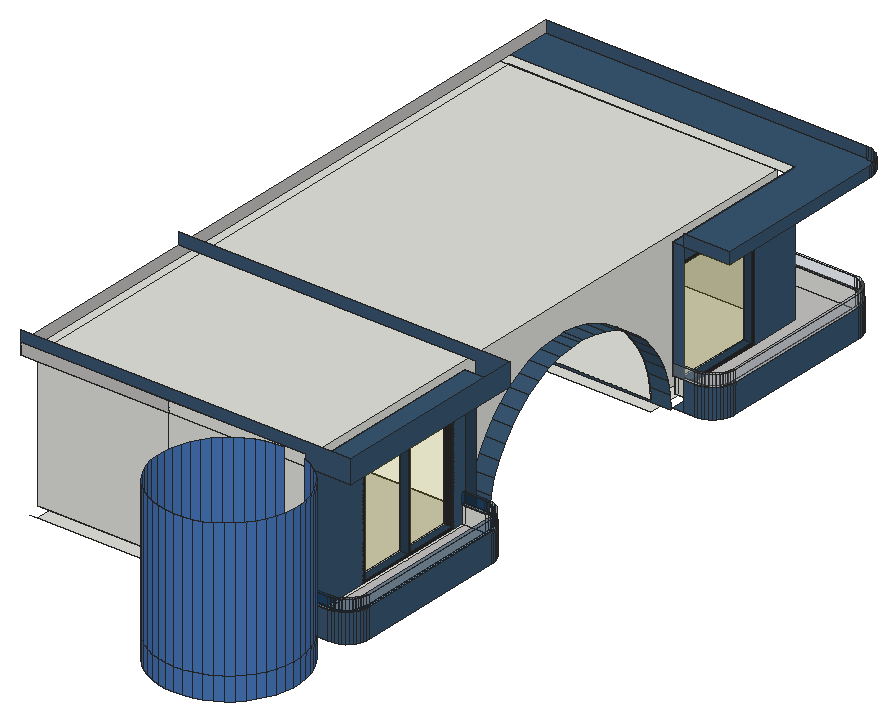
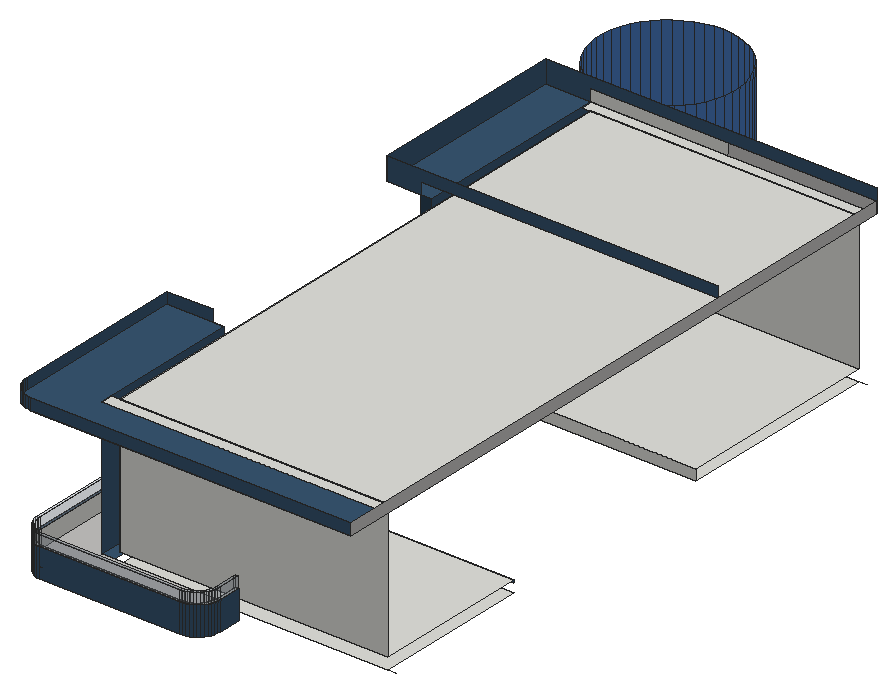
# SketchUp Ruby script. Lengths in inches.
U = 1.inch
M = Sketchup.active_model
def pt(a) = Geom::Point3d.new(a.map { |v| v * U })
def face(e, loops, mat)
  f = e.add_face(loops[0].map { |a| pt(a) })
  loops[1..].each { |l| e.add_face(l.map { |a| pt(a) }).erase! }
  f.material = f.back_material = mat if mat
  f
end
# faces: each face lists its corners as indices into pts; further lists are holes
def faces(e, pts, list, mat = nil) = list.each { |f| face(e, (f[0].is_a?(Array) ? f : [f]).map { |l| l.map { |i| pts[i] } }, mat) }
# xy, xz, yz: faces in a plane at the given z, y or x. An outline is a flat list of corners, or four numbers for a rectangle; further outlines are holes
def ring(l) = l.size == 4 ? [[l[0], l[1]], [l[2], l[1]], [l[2], l[3]], [l[0], l[3]]] : l.each_slice(2).to_a
def flat(e, list, mat, &to3) = list.each { |f| face(e, (f[0].is_a?(Array) ? f : [f]).map { |l| ring(l).map { |u, v| to3.(u, v) } }, mat) }
def xy(e, z, list, mat = nil) = flat(e, list, mat) { |x, y| [x, y, z] }
def xz(e, y, list, mat = nil) = flat(e, list, mat) { |x, z| [x, y, z] }
def yz(e, x, list, mat = nil) = flat(e, list, mat) { |y, z| [x, y, z] }
def lines(e, pts, list) = list.each { |a, b| e.add_line(pt(pts[a]), pt(pts[b])) }
# prism: a flat outline (further loops are holes) pulled along v
def prism(e, loops, v, mat = nil)
  f = face(e, loops, mat); d = Geom::Vector3d.new(v.map { |x| x * U })
  f.pushpull(f.normal.samedirection?(d) ? d.length : -d.length)
end
def box(e, o, s, mat = nil) = prism(e, [[o, [o[0] + s[0], o[1], o[2]], [o[0] + s[0], o[1] + s[1], o[2]], [o[0], o[1] + s[1], o[2]]]], [0, 0, s[2]], mat)
def at(x, y, z, deg = 0) = Geom::Transformation.translation(pt([x, y, z])) * Geom::Transformation.rotation(ORIGIN, Z_AXIS, deg.degrees)
def axes(o, x, y, z) = Geom::Transformation.new([*x, 0, *y, 0, *z, 0, *pt(o).to_a, 1])
def part(name) = M.definitions.add(name)
# library, detail: a bought-in or finely detailed component or shape, given as its bounding box
def library(name, o, s) = part(name).tap { |d| box(d.entities, o, s) }
def detail(e, o, s) = box(e.add_group.entities, o, s)
def put(e, d, t, mat = nil) = e.add_instance(d, t).tap { |i| i.material = mat if mat }
def group(e, t, mat = nil) = e.add_group.tap { |g| g.transformation = t; g.material = mat if mat }.entities
root = M.entities
M.materials.add("Carpet_01_1K").color = [196, 195, 193]
M.materials.add("Carpet_04_1K").color = [56, 85, 112]
M.materials.add("Carpet_04_1K1").color = [43, 65, 85]
M.materials.add("Glass_Basic_01").color = [186, 175, 28]
M.materials["Glass_Basic_01"].alpha = 0.25
M.materials.add("Glass_Basic_1").color = [0, 47, 91]
M.materials["Glass_Basic_1"].alpha = 0.25
M.materials.add("Glass_Basic_2").color = [161, 173, 186]
M.materials["Glass_Basic_2"].alpha = 0.25
M.materials.add("Glass_Mirror_01").color = [71, 118, 185]
M.materials.add("ThomThom - Buttons2").color = [40, 40, 43]
c1 = part("Group\#1")
prism(c1.entities,[[[0,206.04,0],[0,209.04,0],[24,209.04,0],[24.001,209.04,0],[27.133,208.835,0],[30.212,208.222,0],[33.184,207.213,0],[36,205.825,0],[38.61,204.081,0],[40.971,202.011,0],[43.04,199.65,0],[44.785,197.04,0],[46.173,194.224,0],[47.182,191.252,0],[47.795,188.173,0],[48,185.04,0],[48,24,0],[47.795,20.867,0],[47.182,17.788,0],[46.602,16.08,0],[46.173,14.816,0],[44.785,12,0],[43.04,9.39,0],[40.971,7.029,0],[38.61,4.96,0],[36,3.215,0],[33.184,1.827,0],[30.212,0.818,0],[27.133,0.205,0],[24,0,0],[0,0,0],[0,3,0],[3,3,0],[24,3,0],[26.741,3.18,0],[29.435,3.716,0],[32.036,4.599,0],[34.5,5.814,0],[36.784,7.34,0],[38.849,9.151,0],[40.66,11.216,0],[42.187,13.5,0],[43.401,15.964,0],[44.284,18.565,0],[44.82,21.259,0],[45,24,0],[45,185.04,0],[44.82,187.781,0],[44.284,190.475,0],[43.401,193.076,0],[42.187,195.54,0],[40.66,197.824,0],[38.849,199.889,0],[36.784,201.701,0],[34.5,203.227,0],[32.036,204.442,0],[29.435,205.325,0],[26.741,205.86,0],[24,206.04,0],[3,206.04,0]]],[0,0,12])
c2 = part("Group\#2")
prism(c2.entities,[[[147,3,0],[168,3,0],[170.74,3.18,0],[173.44,3.72,0],[176.04,4.6,0],[178.5,5.8125,0],[180.78,7.34,0],[182.85,9.15,0],[184.66,11.22,0],[186.1875,13.5,0],[187.4,15.96,0],[188.28,18.56,0],[188.82,21.26,0],[189,24,0],[189,184.94,0],[188.8125,187.78,0],[188.28,190.47,0],[187.4,193.07,0],[186.18,195.54,0],[184.66,197.82,0],[182.84,199.88,0],[180.78,201.7,0],[178.5,203.22,0],[176.03,204.4375,0],[173.43,205.32,0],[171.01,205.8,0],[24,205.8,0],[21.26,205.62,0],[18.56,205.08,0],[15.96,204.2,0],[13.5,202.99,0],[11.22,201.46,0],[9.15,199.65,0],[7.34,197.58,0],[5.8125,195.3,0],[4.6,192.84,0],[3.72,190.24,0],[3.18,187.54,0],[3,184.8,0],[3,163.8,0],[3,160.8,0],[0,160.8,0],[0,184.8,0],[0.21,187.93,0],[0.82,191.01,0],[1.83,193.98,0],[3.22,196.8,0],[4.96,199.41,0],[7.03,201.77,0],[9.39,203.84,0],[12,205.58,0],[14.82,206.97,0],[17.79,207.98,0],[20.87,208.59,0],[24,208.8,0],[171.31,208.8,0],[174.21,208.22,0],[177.18,207.21,0],[180,205.82,0],[182.61,204.08,0],[184.97,202.01,0],[187.04,199.65,0],[188.78,197.04,0],[190.17,194.22,0],[191.18,191.25,0],[191.79,188.17,0],[192,185.04,0],[192,24,0],[191.79,20.87,0],[191.18,17.79,0],[190.17,14.82,0],[188.78,12,0],[187.04,9.39,0],[184.97,7.03,0],[182.61,4.96,0],[180,3.22,0],[177.18,1.83,0],[174.21,0.82,0],[171.13,0.21,0],[168,0,0],[144,0,0],[144,3,0]]],[0,0,12])
xy(root,1230,[[39.57,167.5625,321.57,381.51],[39.57,620.85,321.57,786.64]])
xy(root,1230,[[330.57,155.5,330.57,364.54,354.57,364.54,357.71,364.34,360.79,363.72,363.76,362.71,366.57,361.33,369.19,359.58,371.55,357.51,373.62,355.15,375.36,352.54,376.75,349.73,377.76,346.75,378.37,343.67,378.57,340.54,378.57,179.5,378.37,176.37,377.76,173.29,376.75,170.32,375.36,167.5,373.62,164.89,371.55,162.53,369.19,160.46,366.57,158.72,363.76,157.33,360.79,156.32,357.71,155.71,354.57,155.5],[330.57,637.9,330.57,798.7,186.57,798.7,186.57,822.7,186.78,825.83,187.39,828.91,188.4,831.89,189.79,834.7,191.53,837.3125,193.6,839.67,195.96,841.74,198.57,843.49,201.39,844.875,204.36,845.88,207.44,846.5,210.57,846.7,357.88,846.7,360.79,846.12,363.76,845.11,366.57,843.73,369.19,841.98,371.55,839.91,373.62,837.55,375.36,834.94,376.75,832.125,377.76,829.15,378.37,826.07,378.57,822.94,378.57,661.9,378.37,658.77,377.76,655.6875,376.75,652.72,375.36,649.9,373.62,647.29,371.55,644.93,369.19,642.86,366.57,641.12,363.76,639.73,360.79,638.72,357.71,638.11,354.57,637.9]],"Carpet_04_1K")
xy(root,1242,[[330.57,158.5,333.57,361.54],[39.57,167.5625,321.57,381.59],[39.57,620.93,321.57,786.64]])
xy(root,1242,[[333.57,158.5,354.57,158.5,357.32,158.68,360.01,159.22,362.61,160.1,365.07,161.31,367.36,162.84,369.42,164.65,371.24,166.72,372.76,169,373.98,171.46,374.86,174.07,375.4,176.76,375.57,179.5,375.57,340.54,375.4,343.28,374.86,345.98,373.98,348.58,372.76,351.04,371.24,353.33,369.42,355.39,367.36,357.2,365.07,358.73,362.61,359.94,360.01,360.83,357.32,361.36,354.57,361.54,333.57,361.54],[330.57,640.9,354.57,640.9,357.32,641.08,360.01,641.62,362.61,642.5,365.07,643.71,367.36,645.24,369.42,647.05,371.24,649.12,372.76,651.4,373.98,653.86,374.86,656.47,375.4,659.16,375.57,661.9,375.57,822.84,375.39,825.68,374.85,828.375,373.97,830.97,372.76,833.4375,371.23,835.72,369.42,837.79,367.36,839.6,365.07,841.12,362.61,842.34,360.01,843.22,357.59,843.7,210.57,843.7,207.83,843.52,205.14,842.99,202.54,842.1,200.07,840.89,197.79,839.36,195.73,837.55,193.91,835.48,192.39,833.2,191.17,830.74,190.29,828.14,189.75,825.44,189.57,822.7,189.57,798.7,330.57,798.7]],"Carpet_01_1K")
xy(root,1244,[[321.57,233.15,330.57,291.15],[321.57,293.15,330.57,349.15]],"Carpet_04_1K1")
xy(root,1245,[[321.57,652.9,330.57,742.9]],"Carpet_04_1K1")
xy(root,1260,[[330.57,155.5,354.57,155.5,357.71,155.71,360.79,156.32,363.76,157.33,366.57,158.72,369.19,160.46,371.55,162.53,373.62,164.89,375.36,167.5,376.75,170.32,377.76,173.29,378.37,176.37,378.57,179.5,378.57,340.54,378.37,343.67,377.76,346.75,376.75,349.73,375.36,352.54,373.62,355.15,371.55,357.51,369.19,359.58,366.57,361.33,363.76,362.71,360.79,363.72,357.71,364.34,354.57,364.54,330.57,364.54,330.57,361.54,354.57,361.54,357.32,361.36,360.01,360.83,362.61,359.94,365.07,358.73,367.36,357.2,369.42,355.39,371.24,353.33,372.76,351.04,373.98,348.58,374.86,345.98,375.4,343.28,375.57,340.54,375.57,179.5,375.4,176.76,374.86,174.07,373.98,171.46,372.76,169,371.24,166.72,369.42,164.65,367.36,162.84,365.07,161.31,362.61,160.1,360.01,159.22,357.32,158.68,354.57,158.5,330.57,158.5]])
xy(root,1359,[[321.57,652.9,330.57,742.9]])
xy(root,1366,[[321.57,233.15,330.57,291.15],[321.57,293.15,330.57,349.15]])
xy(root,1386,[[30.57,155.5,330.57,167.5625],[30.57,167.5625,39.57,786.64],[39.57,167.5625,321.57,786.64],[30.57,786.64,330.57,798.7]])
xy(root,1386,[[330.57,155.5,378.57,364.54],[330.57,637.9,330.57,798.7,30.57,798.7,30.57,846.7,366.57,846.7,369.71,846.5,372.79,845.88,375.76,844.875,378.57,843.49,381.19,841.74,383.55,839.67,385.62,837.3125,387.36,834.7,388.75,831.89,389.76,828.91,390.37,825.83,390.57,822.7,390.57,637.9]],"Carpet_04_1K")
xz(root,155.5,[[186.57,1230,330.57,1242],[186.57,1242,330.57,1386],[186.57,1386,330.57,1398]])
xz(root,155.5,[[30.57,1386,186.57,1398]],"Carpet_01_1K")
xz(root,155.5,[[330.57,1230,354.57,1260],[330.57,1386,378.57,1386,378.57,1410,30.57,1410,30.57,1398,330.57,1398]],"Carpet_04_1K")
xz(root,158.5,[[330.57,1242,333.57,1260],[333.57,1242,354.57,1260]])
xz(root,167.5625,[[39.57,1242,321.57,1386]])
xz(root,233.15,[[321.57,1244,330.57,1366]],"ThomThom - Buttons2")
xz(root,291.15,[[321.57,1244,330.57,1366]],"Carpet_04_1K1")
xz(root,293.15,[[321.57,1244,330.57,1366]],"ThomThom - Buttons2")
xz(root,349.15,[[321.57,1244,330.57,1366]],"ThomThom - Buttons2")
xz(root,361.54,[[330.57,1242,333.57,1260],[333.57,1242,354.57,1260]])
xz(root,364.54,[[342.57,1230,354.57,1260],[342.57,1386,342.57,1398,30.57,1398,30.57,1410,378.57,1410,378.57,1386]],"Carpet_04_1K")
xz(root,364.54,[[330.57,1260,342.57,1386]],"Carpet_04_1K1")
xz(root,637.9,[[342.57,1230,354.57,1260],[330.57,1260,342.57,1386],[342.57,1386,390.57,1398]],"Carpet_04_1K")
xz(root,640.9,[[330.57,1242,333.57,1260],[333.57,1242,354.57,1260]])
xz(root,652.9,[[321.57,1245,330.57,1359]])
xz(root,742.9,[[321.57,1245,330.57,1359]],"Carpet_04_1K1")
xz(root,786.64,[[39.57,1242,321.57,1386]])
xz(root,843.7,[[210.57,1242,357.59,1260]])
xz(root,846.7,[[210.57,1230,357.88,1260],[30.57,1386,366.57,1398]],"Carpet_04_1K")
yz(root,30.57,[[155.5,1386,846.7,1398]],"Carpet_01_1K")
yz(root,186.57,[[149.51,1230,155.5,1242]],"Carpet_01_1K")
yz(root,186.57,[[798.7,1230,822.7,1260]],"Carpet_04_1K")
yz(root,189.57,[[798.7,1242,801.7,1260],[801.7,1242,822.7,1260]])
yz(root,236.92,[[77.22,1230,86.26,1254],[77.22,1254,86.26,1398]],"Glass_Mirror_01")
yz(root,321.57,[[381.51,1230,381.59,1242,381.27,1232.66],[[167.5625,1242,167.5625,1386,786.64,1386,786.64,1242,620.93,1242,619.8125,1254.34,616.58,1269.0625,611.52,1283.26,604.73,1296.71,596.3,1309.21,586.38,1320.55,575.11,1330.55,562.68,1339.07,549.28,1345.96,535.12,1351.11,520.42,1354.45,505.42,1355.93,501.22,1355.81,490.36,1355.51,475.47,1353.2,460.98,1349.05,447.13,1343.12,434.13,1335.49,422.1875,1326.3,411.49,1315.68,402.22,1303.81,394.5,1290.86,388.46,1277.06,384.21,1262.6,381.8,1247.72,381.59,1242],[652.9,1245,742.9,1359],[233.15,1244,291.15,1366],[293.15,1244,349.15,1366]]])
yz(root,321.57,[[233.15,1244,291.15,1366],[293.15,1244,349.15,1366],[652.9,1245,742.9,1359]],"Glass_Basic_01")
yz(root,330.57,[[158.5,1242,231.15,1242,231.15,1368,351.15,1368,351.15,1242,361.54,1242,361.54,1260,364.54,1260,364.54,1386,155.5,1386,155.5,1260,158.5,1260],[640.9,1242,649.9,1242,649.9,1362,745.9,1362,745.9,1242,798.7,1242,798.7,1386,637.9,1386,637.9,1260,640.9,1260]],"Carpet_04_1K")
yz(root,330.57,[[[231.15,1242,351.15,1368],[233.15,1244,233.15,1366,349.15,1366,349.15,1244,293.15,1244,293.15,1366,291.15,1366,291.15,1244]],[[649.9,1242,745.9,1362],[652.9,1245,742.9,1359]]],"ThomThom - Buttons2")
yz(root,375.57,[[179.5,1242,340.54,1260],[661.9,1242,822.84,1260]])
yz(root,378.57,[[179.5,1230,340.54,1260],[661.9,1230,822.94,1260],[155.5,1386,364.54,1410]],"Carpet_04_1K")
yz(root,380.64,[[77.22,1230,86.26,1254],[77.22,1254,86.26,1398]],"Glass_Mirror_01")
yz(root,390.57,[[637.9,1386,822.7,1398]],"Carpet_04_1K")
p = [[299.76,10.31,1254],[299.76,10.31,1230],[308.78,9.74,1230],[308.78,9.74,1254],[317.8,10.31,1230],[317.8,10.31,1254],
  [290.875,12,1254],[290.875,12,1230],[326.6875,12,1230],[326.6875,12,1254],[282.28,14.79,1254],[282.28,14.79,1230],
  [335.29,14.79,1230],[335.29,14.79,1254],[274.09,18.64,1254],[274.09,18.64,1230],[343.47,18.64,1230],[343.47,18.64,1254],
  [266.46,23.49,1254],[266.46,23.49,1230],[351.1,23.49,1230],[351.1,23.49,1254],[259.49,29.25,1254],[259.49,29.25,1230],
  [358.07,29.25,1230],[358.07,29.25,1254],[253.3,35.84,1254],[253.3,35.84,1230],[364.26,35.84,1230],[364.26,35.84,1254],
  [247.99,43.16,1254],[247.99,43.16,1230],[369.57,43.16,1230],[369.57,43.16,1254],[243.63,51.08,1254],[243.63,51.08,1230],
  [373.93,51.08,1230],[373.93,51.08,1254],[240.3,59.49,1254],[240.3,59.49,1230],[377.26,59.49,1230],[377.26,59.49,1254],
  [238.06,68.25,1254],[238.06,68.25,1230],[379.51,68.25,1230],[379.51,68.25,1254],[236.92,77.22,1254],[236.92,77.22,1230],
  [380.64,77.22,1230],[380.64,77.22,1254],[238.06,95.23,1254],[238.06,95.23,1230],[236.92,86.26,1230],[236.92,86.26,1254],
  [380.64,86.26,1254],[380.64,86.26,1230],[379.51,95.23,1230],[379.51,95.23,1254],[240.3,103.99,1254],[240.3,103.99,1230],
  [377.26,103.99,1230],[377.26,103.99,1254],[243.63,112.39,1254],[243.63,112.39,1230],[373.93,112.39,1230],[373.93,112.39,1254],
  [247.99,120.32,1254],[247.99,120.32,1230],[369.57,120.32,1230],[369.57,120.32,1254],[253.3,127.63,1254],[253.3,127.63,1230],
  [364.26,127.63,1230],[364.26,127.63,1254],[259.49,134.22,1254],[259.49,134.22,1230],[358.07,134.22,1230],[358.07,134.22,1254],
  [266.46,139.99,1254],[266.46,139.99,1230],[351.1,139.99,1230],[351.1,139.99,1254],[274.09,144.83,1254],[274.09,144.83,1230],
  [343.47,144.83,1230],[343.47,144.83,1254],[282.28,148.68,1254],[282.28,148.68,1230],[335.29,148.68,1230],[335.29,148.68,1254],
  [290.875,151.48,1254],[290.875,151.48,1230],[299.76,153.17,1254],[299.76,153.17,1230],[308.78,153.74,1254],[308.78,153.74,1230],
  [357.71,155.71,1230],[357.71,155.71,1260],[354.57,155.5,1260],[354.57,155.5,1230],[360.79,156.32,1230],[360.79,156.32,1260],
  [363.76,157.33,1230],[363.76,157.33,1260],[366.57,158.72,1230],[366.57,158.72,1260],[369.19,160.46,1230],[369.19,160.46,1260],
  [371.55,162.53,1230],[371.55,162.53,1260],[373.62,164.89,1230],[373.62,164.89,1260],[375.36,167.5,1230],[375.36,167.5,1260],
  [376.75,170.32,1230],[376.75,170.32,1260],[377.76,173.29,1230],[377.76,173.29,1260],[378.37,176.37,1230],[378.37,176.37,1260],
  [378.57,179.5,1230],[378.57,179.5,1260],[378.37,343.67,1230],[378.37,343.67,1260],[378.57,340.54,1260],[378.57,340.54,1230],
  [377.76,346.75,1230],[377.76,346.75,1260],[376.75,349.73,1230],[376.75,349.73,1260],[375.36,352.54,1230],[375.36,352.54,1260],
  [373.62,355.15,1230],[373.62,355.15,1260],[371.55,357.51,1230],[371.55,357.51,1260],[369.19,359.58,1230],[369.19,359.58,1260],
  [366.57,361.33,1230],[366.57,361.33,1260],[363.76,362.71,1230],[363.76,362.71,1260],[360.79,363.72,1230],[360.79,363.72,1260],
  [357.71,364.34,1230],[357.71,364.34,1260],[354.57,364.54,1230],[354.57,364.54,1260],[321.57,381.59,1242],[321.57,381.51,1230],
  [39.57,381.51,1230],[39.57,381.59,1242],[357.71,638.11,1230],[357.71,638.11,1260],[354.57,637.9,1260],[354.57,637.9,1230],
  [360.79,638.72,1230],[360.79,638.72,1260],[363.76,639.73,1230],[363.76,639.73,1260],[366.57,641.12,1230],[366.57,641.12,1260],
  [369.19,642.86,1230],[369.19,642.86,1260],[371.55,644.93,1230],[371.55,644.93,1260],[373.62,647.29,1230],[373.62,647.29,1260],
  [375.36,649.9,1230],[375.36,649.9,1260],[376.75,652.72,1230],[376.75,652.72,1260],[377.76,655.6875,1230],[377.76,655.6875,1260],
  [378.37,658.77,1230],[378.37,658.77,1260],[378.57,661.9,1230],[378.57,661.9,1260],[186.57,822.7,1230],[186.57,822.7,1260],
  [186.78,825.83,1260],[186.78,825.83,1230],[378.37,826.07,1230],[378.37,826.07,1260],[378.57,822.94,1260],[378.57,822.94,1230],
  [187.39,828.91,1260],[187.39,828.91,1230],[377.76,829.15,1230],[377.76,829.15,1260],[188.4,831.89,1260],[188.4,831.89,1230],
  [376.75,832.125,1230],[376.75,832.125,1260],[189.79,834.7,1260],[189.79,834.7,1230],[375.36,834.94,1230],[375.36,834.94,1260],
  [191.53,837.3125,1260],[191.53,837.3125,1230],[373.62,837.55,1230],[373.62,837.55,1260],[193.6,839.67,1260],[193.6,839.67,1230],
  [371.55,839.91,1230],[371.55,839.91,1260],[195.96,841.74,1260],[195.96,841.74,1230],[369.19,841.98,1230],[369.19,841.98,1260],
  [198.57,843.49,1260],[198.57,843.49,1230],[366.57,843.73,1230],[366.57,843.73,1260],[201.39,844.875,1260],[201.39,844.875,1230],
  [363.76,845.11,1230],[363.76,845.11,1260],[204.36,845.88,1260],[204.36,845.88,1230],[360.79,846.12,1230],[360.79,846.12,1260],
  [207.44,846.5,1260],[207.44,846.5,1230],[357.88,846.7,1242],[357.88,846.7,1260],[357.88,846.7,1230],[210.57,846.7,1260],
  [210.57,846.7,1230],[321.57,381.8,1247.72],[342.57,381.8,1247.72],[342.57,381.27,1232.66],[321.57,381.27,1232.66],[39.57,621.17,1239.34],
  [342.57,621.17,1239.34],[342.57,619.8125,1254.34],[321.57,619.8125,1254.34],[321.57,620.93,1242],[39.57,620.93,1242],[357.32,158.68,1242],
  [354.57,158.5,1242],[354.57,158.5,1260],[357.32,158.68,1260],[360.01,159.22,1242],[360.01,159.22,1260],[362.61,160.1,1242],
  [362.61,160.1,1260],[365.07,161.31,1242],[365.07,161.31,1260],[367.36,162.84,1242],[367.36,162.84,1260],[369.42,164.65,1242],
  [369.42,164.65,1260],[371.24,166.72,1242],[371.24,166.72,1260],[372.76,169,1242],[372.76,169,1260],[373.98,171.46,1242],
  [373.98,171.46,1260],[374.86,174.07,1242],[374.86,174.07,1260],[375.4,176.76,1242],[375.4,176.76,1260],[375.57,179.5,1242],
  [375.57,179.5,1260],[375.4,343.28,1242],[375.57,340.54,1242],[375.57,340.54,1260],[375.4,343.28,1260],[374.86,345.98,1242],
  [374.86,345.98,1260],[373.98,348.58,1242],[373.98,348.58,1260],[372.76,351.04,1242],[372.76,351.04,1260],[371.24,353.33,1242],
  [371.24,353.33,1260],[369.42,355.39,1242],[369.42,355.39,1260],[367.36,357.2,1242],[367.36,357.2,1260],[365.07,358.73,1242],
  [365.07,358.73,1260],[362.61,359.94,1242],[362.61,359.94,1260],[360.01,360.83,1242],[360.01,360.83,1260],[357.32,361.36,1242],
  [357.32,361.36,1260],[354.57,361.54,1242],[354.57,361.54,1260],[357.32,641.08,1242],[354.57,640.9,1242],[354.57,640.9,1260],
  [357.32,641.08,1260],[360.01,641.62,1242],[360.01,641.62,1260],[362.61,642.5,1242],[362.61,642.5,1260],[365.07,643.71,1242],
  [365.07,643.71,1260],[367.36,645.24,1242],[367.36,645.24,1260],[369.42,647.05,1242],[369.42,647.05,1260],[371.24,649.12,1242],
  [371.24,649.12,1260],[372.76,651.4,1242],[372.76,651.4,1260],[373.98,653.86,1242],[373.98,653.86,1260],[374.86,656.47,1242],
  [374.86,656.47,1260],[375.4,659.16,1242],[375.4,659.16,1260],[375.57,661.9,1242],[375.57,661.9,1260],[189.57,822.7,1242],
  [189.75,825.44,1242],[189.75,825.44,1260],[189.57,822.7,1260],[375.39,825.68,1242],[375.57,822.84,1242],[375.57,822.84,1260],
  [375.39,825.68,1260],[190.29,828.14,1242],[190.29,828.14,1260],[374.85,828.375,1242],[374.85,828.375,1260],[191.17,830.74,1242],
  [191.17,830.74,1260],[373.97,830.97,1242],[373.97,830.97,1260],[192.39,833.2,1242],[192.39,833.2,1260],[372.76,833.4375,1242],
  [372.76,833.4375,1260],[193.91,835.48,1242],[193.91,835.48,1260],[371.23,835.72,1242],[371.23,835.72,1260],[195.73,837.55,1242],
  [195.73,837.55,1260],[369.42,837.79,1242],[369.42,837.79,1260],[197.79,839.36,1242],[197.79,839.36,1260],[367.36,839.6,1242],
  [367.36,839.6,1260],[200.07,840.89,1242],[200.07,840.89,1260],[365.07,841.12,1242],[365.07,841.12,1260],[202.54,842.1,1242],
  [202.54,842.1,1260],[362.61,842.34,1242],[362.61,842.34,1260],[205.14,842.99,1242],[205.14,842.99,1260],[360.01,843.22,1242],
  [360.01,843.22,1260],[207.83,843.52,1242],[207.83,843.52,1260],[357.59,843.7,1242],[357.59,843.7,1260],[210.57,843.7,1242],
  [210.57,843.7,1260],[321.57,384.21,1262.6],[342.57,384.21,1262.6],[299.76,10.31,1398],[308.78,9.74,1398],[317.8,10.31,1398],
  [290.875,12,1398],[326.6875,12,1398],[282.28,14.79,1398],[335.29,14.79,1398],[274.09,18.64,1398],[343.47,18.64,1398],
  [266.46,23.49,1398],[351.1,23.49,1398],[259.49,29.25,1398],[358.07,29.25,1398],[253.3,35.84,1398],[364.26,35.84,1398],
  [247.99,43.16,1398],[369.57,43.16,1398],[243.63,51.08,1398],[373.93,51.08,1398],[240.3,59.49,1398],[377.26,59.49,1398],
  [238.06,68.25,1398],[379.51,68.25,1398],[236.92,77.22,1398],[380.64,77.22,1398],[238.06,95.23,1398],[236.92,86.26,1398],
  [380.64,86.26,1398],[379.51,95.23,1398],[240.3,103.99,1398],[377.26,103.99,1398],[243.63,112.39,1398],[373.93,112.39,1398],
  [247.99,120.32,1398],[369.57,120.32,1398],[253.3,127.63,1398],[364.26,127.63,1398],[259.49,134.22,1398],[358.07,134.22,1398],
  [266.46,139.99,1398],[351.1,139.99,1398],[274.09,144.83,1398],[343.47,144.83,1398],[282.28,148.68,1398],[335.29,148.68,1398],
  [290.875,151.48,1398],[299.76,153.17,1398],[308.78,153.74,1398],[342.57,616.58,1269.0625],[321.57,616.58,1269.0625],[321.57,388.46,1277.06],
  [342.57,388.46,1277.06],[342.57,611.52,1283.26],[321.57,611.52,1283.26],[321.57,394.5,1290.86],[342.57,394.5,1290.86],[342.57,604.73,1296.71],
  [321.57,604.73,1296.71],[321.57,402.22,1303.81],[342.57,402.22,1303.81],[342.57,596.3,1309.21],[321.57,596.3,1309.21],[321.57,411.49,1315.68],
  [342.57,411.49,1315.68],[342.57,586.38,1320.55],[321.57,586.38,1320.55],[321.57,422.1875,1326.3],[342.57,422.1875,1326.3],[342.57,575.11,1330.55],
  [321.57,575.11,1330.55],[321.57,434.13,1335.49],[342.57,434.13,1335.49],[342.57,562.68,1339.07],[321.57,562.68,1339.07],[321.57,447.13,1343.12],
  [342.57,447.13,1343.12],[342.57,549.28,1345.96],[321.57,549.28,1345.96],[321.57,460.98,1349.05],[342.57,460.98,1349.05],[342.57,535.12,1351.11],
  [321.57,535.12,1351.11],[321.57,475.47,1353.2],[342.57,475.47,1353.2],[342.57,520.42,1354.45],[321.57,520.42,1354.45],[321.57,490.36,1355.51],
  [342.57,490.36,1355.51],[342.57,505.42,1355.93],[321.57,505.42,1355.93],[321.57,501.22,1355.81],[342.57,501.22,1355.81],[390.37,825.83,1398],
  [390.57,822.7,1398],[390.57,822.7,1386],[390.37,825.83,1386],[389.76,828.91,1398],[389.76,828.91,1386],[388.75,831.89,1398],
  [388.75,831.89,1386],[387.36,834.7,1398],[387.36,834.7,1386],[385.62,837.3125,1398],[385.62,837.3125,1386],[383.55,839.67,1398],
  [383.55,839.67,1386],[381.19,841.74,1398],[381.19,841.74,1386],[378.57,843.49,1398],[378.57,843.49,1386],[375.76,844.875,1398],
  [375.76,844.875,1386],[372.79,845.88,1398],[372.79,845.88,1386],[369.71,846.5,1398],[369.71,846.5,1386],[366.57,846.7,1398],
  [366.57,846.7,1386],[321.57,786.64,1230],[330.57,786.64,1230],[39.57,786.64,1230],[30.57,786.64,1230],[39.57,167.5625,1230],
  [30.57,167.5625,1230],[321.57,167.5625,1230],[330.57,167.5625,1230],[357.71,846.74,1242],[354.57,846.94,1242],[330.57,150.21,1254],
  [330.57,150.21,1230]]
faces(root,p,[[0,1,2,3],[3,2,4,5],[6,7,1,0],[5,4,8,9],[10,11,7,6],[9,8,12,13],[14,15,11,10],[13,12,16,17],
  [18,19,15,14],[17,16,20,21],[22,23,19,18],[21,20,24,25],[26,27,23,22],[25,24,28,29],[30,31,27,26],[29,28,32,33],
  [34,35,31,30],[33,32,36,37],[38,39,35,34],[37,36,40,41],[42,43,39,38],[41,40,44,45],[46,47,43,42],[45,44,48,49],
  [50,51,52,53],[54,55,56,57],[58,59,51,50],[57,56,60,61],[62,63,59,58],[61,60,64,65],[66,67,63,62],[65,64,68,69],
  [70,71,67,66],[69,68,72,73],[74,75,71,70],[73,72,76,77],[78,79,75,74],[77,76,80,81],[82,83,79,78],[81,80,84,85],
  [86,87,83,82],[85,84,88,89],[90,91,87,86],[92,93,91,90],[94,95,93,92],[369,0,3,370],[370,3,5,371],[372,6,0,369],
  [371,5,9,373],[374,10,6,372],[373,9,13,375],[376,14,10,374],[375,13,17,377],[378,18,14,376],[377,17,21,379],[380,22,18,378],
  [379,21,25,381],[382,26,22,380],[381,25,29,383],[384,30,26,382],[383,29,33,385],[386,34,30,384],[385,33,37,387],[388,38,34,386],
  [387,37,41,389],[390,42,38,388],[389,41,45,391],[392,46,42,390],[391,45,49,393],[394,50,53,395],[396,54,57,397],[398,58,50,394],
  [397,57,61,399],[400,62,58,398],[399,61,65,401],[402,66,62,400],[401,65,69,403],[404,70,66,402],[403,69,73,405],[406,74,70,404],
  [405,73,77,407],[408,78,74,406],[407,77,81,409],[410,82,78,408],[409,81,85,411],[412,86,82,410],[411,85,89,413],[414,90,86,412],
  [415,92,90,414],[416,94,92,415]],"Glass_Mirror_01")
faces(root,p,[[96,97,98,99],[100,101,97,96],[102,103,101,100],[104,105,103,102],[106,107,105,104],[108,109,107,106],[110,111,109,108],[112,113,111,110],
  [114,115,113,112],[116,117,115,114],[118,119,117,116],[120,121,119,118],[122,123,124,125],[126,127,123,122],[128,129,127,126],[130,131,129,128],
  [132,133,131,130],[134,135,133,132],[136,137,135,134],[138,139,137,136],[140,141,139,138],[142,143,141,140],[144,145,143,142],[146,147,145,144],
  [152,153,154,155],[156,157,153,152],[158,159,157,156],[160,161,159,158],[162,163,161,160],[164,165,163,162],[166,167,165,164],[168,169,167,166],
  [170,171,169,168],[172,173,171,170],[174,175,173,172],[176,177,175,174],[178,179,180,181],[182,183,184,185],[181,180,186,187],[188,189,183,182],
  [187,186,190,191],[192,193,189,188],[191,190,194,195],[196,197,193,192],[195,194,198,199],[200,201,197,196],[199,198,202,203],[204,205,201,200],
  [203,202,206,207],[208,209,205,204],[207,206,210,211],[212,213,209,208],[211,210,214,215],[216,217,213,212],[215,214,218,219],[220,221,217,216],
  [219,218,222,223],[224,225,221,220,226],[223,222,227,228],[229,230,231,232,148],[233,234,235,236,237,238],[367,368,230,229],[236,235,417,418],[419,420,368,367],
  [418,417,421,422],[423,424,420,419],[422,421,425,426],[427,428,424,423],[426,425,429,430],[431,432,428,427],[430,429,433,434],[435,436,432,431],
  [434,433,437,438],[439,440,436,435],[438,437,441,442],[443,444,440,439],[442,441,445,446],[447,448,444,443],[446,445,449,450],[451,452,448,447],
  [450,449,453,454],[455,456,452,451],[454,453,457,458],[459,460,456,455],[458,457,460,459],[461,462,463,464],[465,461,464,466],[467,465,466,468],
  [469,467,468,470],[471,469,470,472],[473,471,472,474],[475,473,474,476],[477,475,476,478],[479,477,478,480],[481,479,480,482],[483,481,482,484],
  [485,483,484,486]],"Carpet_04_1K")
faces(root,p,[[148,149,150,151],[239,240,241,242],[243,239,242,244],[245,243,244,246],[247,245,246,248],[249,247,248,250],[251,249,250,252],[253,251,252,254],
  [255,253,254,256],[257,255,256,258],[259,257,258,260],[261,259,260,262],[263,261,262,264],[265,266,267,268],[269,265,268,270],[271,269,270,272],
  [273,271,272,274],[275,273,274,276],[277,275,276,278],[279,277,278,280],[281,279,280,282],[283,281,282,284],[285,283,284,286],[287,285,286,288],
  [289,287,288,290],[291,292,293,294],[295,291,294,296],[297,295,296,298],[299,297,298,300],[301,299,300,302],[303,301,302,304],[305,303,304,306],
  [307,305,306,308],[309,307,308,310],[311,309,310,312],[313,311,312,314],[315,313,314,316],[317,318,319,320],[321,322,323,324],[318,325,326,319],
  [327,321,324,328],[325,329,330,326],[331,327,328,332],[329,333,334,330],[335,331,332,336],[333,337,338,334],[339,335,336,340],[337,341,342,338],
  [343,339,340,344],[341,345,346,342],[347,343,344,348],[345,349,350,346],[351,347,348,352],[349,353,354,350],[355,351,352,356],[353,357,358,354],
  [359,355,356,360],[357,361,362,358],[363,359,360,364],[361,365,366,362]])
lines(root,p,[[487,488],[489,490],[491,492],[493,494],[495,496],[224,495],[89,497],[88,498]])
put(root,c1,at(330.57,155.5,1260),"Glass_Basic_1")
put(root,c2,at(186.57,637.9,1260),"Glass_Basic_2")
